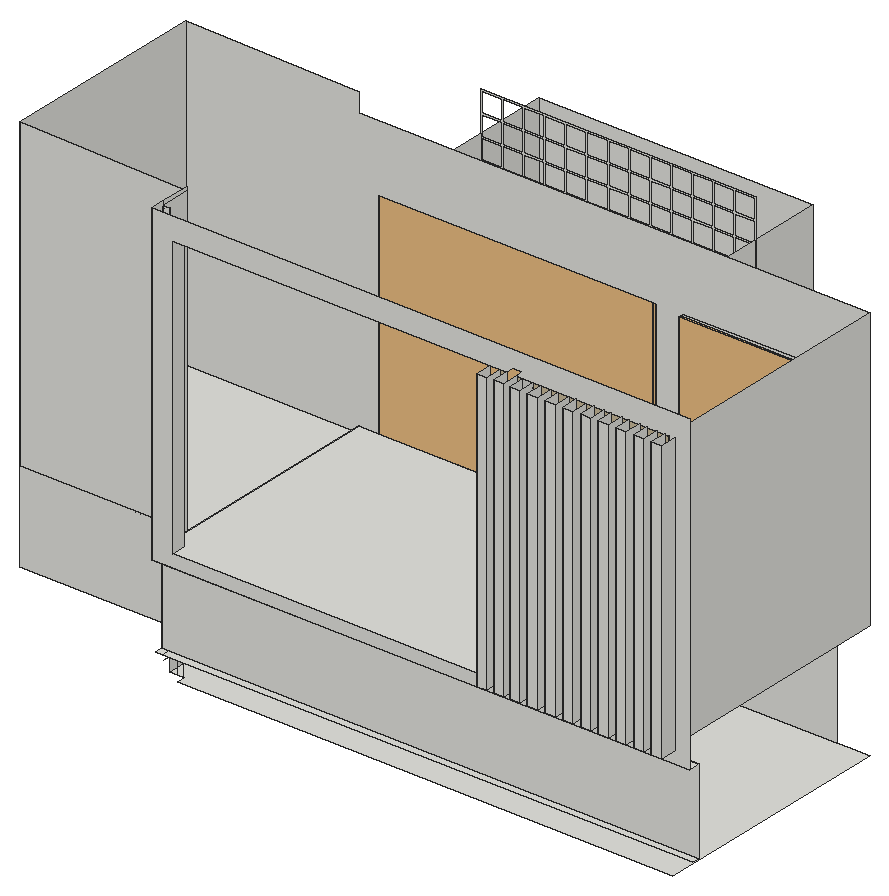
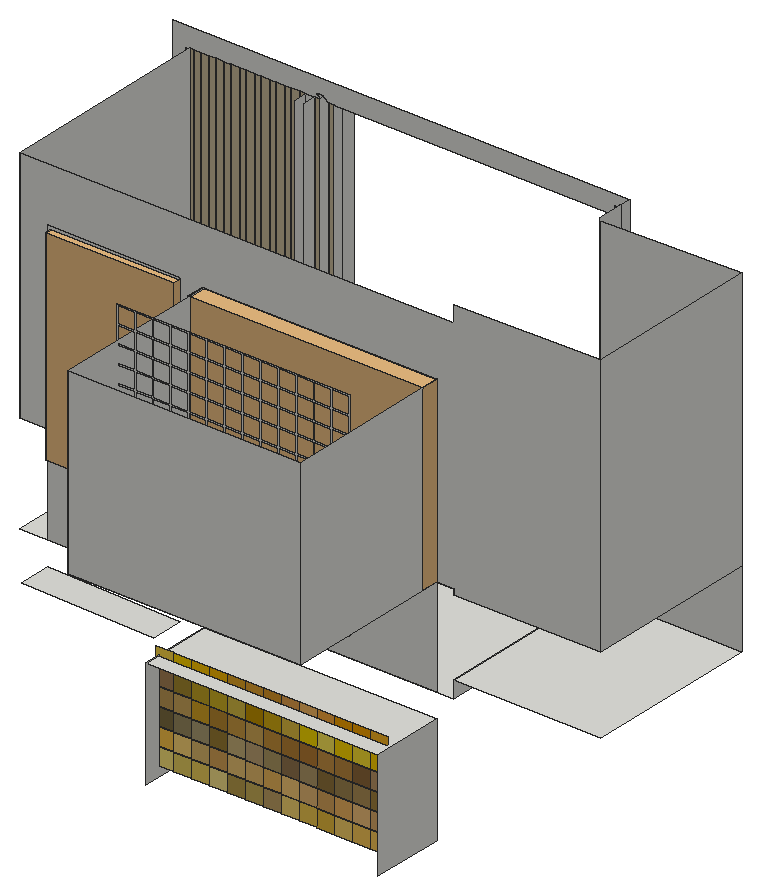
# SketchUp Ruby script. Lengths in inches.
U = 1.inch
M = Sketchup.active_model
def pt(a) = Geom::Point3d.new(a.map { |v| v * U })
def face(e, loops, mat)
  f = e.add_face(loops[0].map { |a| pt(a) })
  loops[1..].each { |l| e.add_face(l.map { |a| pt(a) }).erase! }
  f.material = f.back_material = mat if mat
  f
end
# faces: each face lists its corners as indices into pts; further lists are holes
def faces(e, pts, list, mat = nil) = list.each { |f| face(e, (f[0].is_a?(Array) ? f : [f]).map { |l| l.map { |i| pts[i] } }, mat) }
# xy, xz, yz: faces in a plane at the given z, y or x. An outline is a flat list of corners, or four numbers for a rectangle; further outlines are holes
def ring(l) = l.size == 4 ? [[l[0], l[1]], [l[2], l[1]], [l[2], l[3]], [l[0], l[3]]] : l.each_slice(2).to_a
def flat(e, list, mat, &to3) = list.each { |f| face(e, (f[0].is_a?(Array) ? f : [f]).map { |l| ring(l).map { |u, v| to3.(u, v) } }, mat) }
def xy(e, z, list, mat = nil) = flat(e, list, mat) { |x, y| [x, y, z] }
def xz(e, y, list, mat = nil) = flat(e, list, mat) { |x, z| [x, y, z] }
def yz(e, x, list, mat = nil) = flat(e, list, mat) { |y, z| [x, y, z] }
def lines(e, pts, list) = list.each { |a, b| e.add_line(pt(pts[a]), pt(pts[b])) }
# prism: a flat outline (further loops are holes) pulled along v
def prism(e, loops, v, mat = nil)
  f = face(e, loops, mat); d = Geom::Vector3d.new(v.map { |x| x * U })
  f.pushpull(f.normal.samedirection?(d) ? d.length : -d.length)
end
def box(e, o, s, mat = nil) = prism(e, [[o, [o[0] + s[0], o[1], o[2]], [o[0] + s[0], o[1] + s[1], o[2]], [o[0], o[1] + s[1], o[2]]]], [0, 0, s[2]], mat)
def at(x, y, z, deg = 0) = Geom::Transformation.translation(pt([x, y, z])) * Geom::Transformation.rotation(ORIGIN, Z_AXIS, deg.degrees)
def axes(o, x, y, z) = Geom::Transformation.new([*x, 0, *y, 0, *z, 0, *pt(o).to_a, 1])
def part(name) = M.definitions.add(name)
# library, detail: a bought-in or finely detailed component or shape, given as its bounding box
def library(name, o, s) = part(name).tap { |d| box(d.entities, o, s) }
def detail(e, o, s) = box(e.add_group.entities, o, s)
def put(e, d, t, mat = nil) = e.add_instance(d, t).tap { |i| i.material = mat if mat }
def group(e, t, mat = nil) = e.add_group.tap { |g| g.transformation = t; g.material = mat if mat }.entities
root = M.entities
M.materials.add("SW 0028 Caen Stone").color = [234, 212, 175]
M.materials.add("SW 0043 Peristyle Brass").color = [171, 151, 98]
M.materials.add("SW 2813 Downing Straw").color = [196, 173, 119]
M.materials.add("SW 2814 Rookwood Antique Gold").color = [158, 131, 78]
M.materials.add("SW 2817 Rookwood Amber").color = [185, 135, 62]
M.materials.add("SW 2831 Classical Gold").color = [230, 191, 112]
M.materials.add("SW 2858 Harvest Gold").color = [215, 167, 103]
M.materials.add("SW 6113 Interactive Cream").color = [226, 206, 173]
M.materials.add("SW 6116 Tatami Tan").color = [184, 148, 100]
M.materials.add("SW 6117 Smokey Topaz").color = [164, 127, 83]
M.materials.add("SW 6118 Leather Bound").color = [139, 102, 57]
M.materials.add("SW 6120 Believable Buff").color = [216, 202, 167]
M.materials.add("SW 6123 Baguette").color = [175, 151, 103]
M.materials.add("SW 6127 Ivoire").color = [224, 209, 170]
M.materials.add("SW 6130 Mannered Gold").color = [189, 159, 99]
M.materials.add("SW 6131 Chamois").color = [172, 141, 84]
M.materials.add("SW 6132 Relic Bronze").color = [143, 113, 59]
M.materials.add("SW 6134 Netsuke").color = [220, 210, 175]
M.materials.add("SW 6137 Burlap").color = [170, 155, 114]
M.materials.add("SW 6138 Artifact").color = [151, 136, 95]
M.materials.add("SW 6139 Mossy Gold").color = [124, 107, 64]
M.materials.add("SW 6365 Cachet Cream").color = [240, 220, 183]
M.materials.add("SW 6367 Viva Gold").color = [227, 182, 114]
M.materials.add("SW 6368 Bakelite Gold").color = [212, 162, 89]
M.materials.add("SW 6369 Tassel").color = [195, 143, 67]
M.materials.add("SW 6370 Saucy Gold").color = [179, 122, 51]
M.materials.add("SW 6372 Inviting Ivory").color = [239, 218, 175]
M.materials.add("SW 6374 Torchlight").color = [226, 185, 106]
M.materials.add("SW 6375 Honeycomb").color = [210, 161, 84]
M.materials.add("SW 6376 Gold Coast").color = [195, 143, 57]
M.materials.add("SW 6377 Butterscotch").color = [180, 128, 52]
M.materials.add("SW 6379 Jersey Cream").color = [239, 224, 185]
M.materials.add("SW 6381 Anjou Pear").color = [217, 181, 105]
M.materials.add("SW 6382 Ceremonial Gold").color = [208, 167, 85]
M.materials.add("SW 6383 Golden Rule").color = [199, 153, 65]
M.materials.add("SW 6384 Cut The Mustard").color = [182, 135, 47]
M.materials.add("SW 6387 Compatible Cream").color = [229, 206, 156]
M.materials.add("SW 6389 Butternut").color = [200, 164, 90]
M.materials.add("SW 6390 Bosc Pear").color = [188, 151, 83]
M.materials.add("SW 6391 Gallant Gold").color = [161, 128, 61]
M.materials.add("SW 6393 Convivial Yellow").color = [229, 218, 173]
M.materials.add("SW 6395 Alchemy").color = [197, 171, 86]
M.materials.add("SW 6396 Different Gold").color = [183, 156, 75]
M.materials.add("SW 6397 Nankeen").color = [162, 135, 46]
M.materials.add("SW 6398 Sconce Gold").color = [151, 121, 51]
M.materials.add("SW 6400 Lucent Yellow").color = [223, 213, 164]
M.materials.add("SW 6407 Ancestral Gold").color = [218, 210, 164]
M.materials.add("SW 6661 Papaya").color = [238, 189, 120]
M.materials.add("SW 6662 Summer Day").color = [234, 176, 94]
M.materials.add("SW 6663 Saffron Thread").color = [223, 158, 74]
M.materials.add("SW 6668 Sunrise").color = [242, 197, 116]
M.materials.add("SW 6669 Yarrow").color = [231, 180, 89]
M.materials.add("SW 6670 Gold Crest").color = [221, 159, 46]
M.materials.add("SW 6671 Curry").color = [214, 148, 38]
M.materials.add("SW 6675 Afternoon").color = [248, 209, 116]
M.materials.add("SW 6676 Butterfield").color = [244, 196, 86]
M.materials.add("SW 6677 Goldenrod").color = [244, 196, 86]
M.materials.add("SW 6678 Sunflower").color = [223, 162, 35]
M.materials.add("SW 6682 June Day").color = [242, 210, 111]
M.materials.add("SW 6683 Bee").color = [235, 196, 79]
M.materials.add("SW 6684 Brittlebush").color = [228, 184, 61]
M.materials.add("SW 6685 Trinket").color = [209, 161, 37]
M.materials.add("SW 6689 Overjoy").color = [233, 203, 89]
M.materials.add("SW 6690 Gambol Gold").color = [220, 186, 63]
M.materials.add("SW 6691 Glitzy Gold").color = [208, 168, 18]
M.materials.add("SW 6692 Auric").color = [191, 145, 0]
M.materials.add("SW 6695 Midday").color = [242, 222, 135]
M.materials.add("SW 6696 Quilt Gold").color = [227, 203, 95]
M.materials.add("SW 6697 Nugget").color = [211, 184, 67]
M.materials.add("SW 6698 Kingdom Gold").color = [202, 173, 37]
M.materials.add("SW 6699 Crispy Gold").color = [191, 161, 37]
M.materials.add("SW 6701 Moonraker").color = [234, 231, 176]
M.materials.add("SW 6889 Stirring Orange").color = [243, 181, 96]
M.materials.add("SW 6890 Osage Orange").color = [243, 166, 60]
M.materials.add("SW 6894 Forceful Orange").color = [242, 160, 0]
M.materials.add("SW 6895 Laughing Orange").color = [242, 160, 0]
M.materials.add("SW 6897 Sundance").color = [245, 206, 103]
M.materials.add("SW 6898 Social Butterfly").color = [247, 193, 71]
M.materials.add("SW 6899 Nasturtiumb").color = [246, 178, 33]
M.materials.add("SW 6901 Daffodil").color = [246, 223, 119]
M.materials.add("SW 6902 Decisive Yellow").color = [248, 211, 68]
M.materials.add("SW 6903 Cheerful").color = [250, 208, 0]
M.materials.add("SW 6904 Gusto Gold").color = [245, 181, 0]
M.materials.add("SW 6905 Goldfinch").color = [249, 192, 0]
M.materials.add("SW 6906 Citrus").color = [251, 205, 0]
M.materials.add("SW 6907 Forsythia").color = [251, 210, 0]
M.materials.add("SW 6909 Lemon Twist").color = [248, 227, 86]
M.materials.add("SW 6910 Daisy").color = [246, 220, 49]
M.materials.add("SW 6911 Confident Yellow").color = [245, 214, 0]
M.materials.add("SW 7537 Irish Cream").color = [227, 211, 186]
M.materials.add("SW 7676 Paper Lantern").color = [240, 224, 198]
M.materials.add("SW 7678 Cottage Cream").color = [236, 219, 189]
M.materials.add("SW 7681 Tea Light").color = [246, 227, 194]
M.materials.add("SW 7683 Buff").color = [242, 225, 197]
M.materials.add("SW 7684 Concord Buff").color = [239, 216, 182]
M.materials.add("SW 7686 Hinoki").color = [246, 220, 183]
M.materials.add("SW 7687 August Moon").color = [231, 199, 161]
M.materials.add("SW 7688 Sundew").color = [223, 206, 176]
M.materials.add("SW 7696 Toasted Pine Nut").color = [218, 199, 167]
M.materials.add("SW 7698 Straw Harvest").color = [217, 199, 161]
M.materials.add("SW 7699 Rustic City").color = [188, 160, 113]
M.materials.add("SW 7700 Olde World Gold").color = [145, 116, 76]
M.materials.add("[Quartz Light Brown]").color = [199, 184, 152]
c1 = library("Group6\#1",[-22.44,-5.97,0],[42.52,9.29,84.25])
c2 = library("Glass_door",[70.54,1.5625,0],[78.74,7.87,82.68])
xy(root,1139.55,[[1349.53,376.08,1604.22,455.83]])
xy(root,1165.72,[[1344.39,147.66,1344.39,155.91,1330.95,155.91,1330.95,376.08,1805.83,376.08,1805.83,147.66]])
xy(root,1184.06,[[1324.51,147.66,1330.95,154.6],[1330.95,147.66,1824.45,154.6],[1324.16,154.6,1324.51,155.91],[1324.51,154.6,1330.95,155.91],[1330.44,155.91,1330.44,183.72,1169.07,183.72,1169.07,376.08,1330.95,376.08,1330.95,155.91],
  [1324.51,155.91,1330.44,183.72]])
xy(root,1262.78,[[1324.16,143.16,1824.45,154.6]])
xy(root,1268.3125,[[1324.16,155.91,1324.51,183.72],[1324.51,155.91,1330.44,183.72],[1169.07,183.72,1324.16,376.08],[1324.16,183.72,1330.44,376.08]])
xy(root,1274.1875,[[1638.86,127.85,1648.04,143.16],[1654.29,127.85,1663.98,143.16],[1669.29,127.85,1678.97,143.16],[1343.63,143.16,1669.29,143.16,1669.29,158.47,1678.97,158.47,1678.97,143.16,1805.83,143.16,1805.83,376.08,1330.44,376.08,1330.44,155.91,1343.63,155.91],[1669.29,143.16,1678.97,158.47],
  [1349.53,376.08,1604.22,561.95]])
xz(root,127.85,[[1638.86,1274.1875,1648.04,1534.95],[1654.29,1274.1875,1663.98,1534.95],[1669.29,1274.1875,1678.97,1534.95],[1685.79,1274.1875,1695.47,1534.95],[1702.29,1274.1875,1711.97,1534.95],
  [1718.79,1274.1875,1728.47,1534.95],[1735.29,1274.1875,1744.97,1534.95],[1751.79,1274.1875,1761.47,1534.95],[1768.29,1274.1875,1777.97,1534.95],[1784.79,1274.1875,1794.47,1534.95],
  [1801.29,1274.1875,1810.97,1534.95]])
xz(root,143.16,[[[1324.16,1262.78,1824.45,1555.875],[1343.63,1274.1875,1343.63,1534.95,1654.29,1534.95,1659.92,1540.4375,1669.6,1540.4375,1663.98,1534.95,1805.83,1534.95,1805.83,1274.1875]]])
xz(root,143.16,[[1648.04,1274.1875,1654.29,1534.95],[1663.98,1274.1875,1669.29,1534.95],[1678.97,1274.1875,1685.79,1534.95],[1685.79,1274.1875,1695.47,1534.95],[1695.47,1274.1875,1702.29,1534.95],
  [1702.29,1274.1875,1711.97,1534.95],[1711.97,1274.1875,1718.79,1534.95],[1718.79,1274.1875,1728.47,1534.95],[1728.47,1274.1875,1735.29,1534.95],[1735.29,1274.1875,1744.97,1534.95],
  [1744.97,1274.1875,1751.79,1534.95],[1751.79,1274.1875,1761.47,1534.95],[1761.47,1274.1875,1768.29,1534.95],[1768.29,1274.1875,1777.97,1534.95],[1777.97,1274.1875,1784.79,1534.95],
  [1784.79,1274.1875,1794.47,1534.95],[1794.47,1274.1875,1801.29,1534.95],[1801.29,1274.1875,1805.83,1534.95]],"[Quartz Light Brown]")
xz(root,154.6,[[1324.16,1184.06,1824.45,1262.78]])
xz(root,155.91,[[1324.16,1184.06,1324.61,1268.3125],[1324.61,1184.06,1329.57,1268.3125],[1329.57,1184.06,1330.44,1268.3125],[1324.16,1268.3125,1324.51,1555.875],[1324.51,1268.3125,1324.61,1552.52],
  [1324.61,1268.3125,1329.57,1552.52],[1329.57,1268.3125,1329.57,1552.52,1330.44,1552.52,1330.44,1534.95,1337.99,1534.95,1337.99,1274.1875,1330.44,1274.1875,1330.44,1268.3125],[1337.99,1274.1875,1342.94,1534.95],[1342.94,1274.1875,1343.63,1534.95]])
xz(root,183.72,[[1169.07,1184.06,1330.44,1268.3125],[1169.07,1268.3125,1169.07,1555.64,1324.16,1552.64,1324.16,1268.3125],[1324.16,1268.3125,1324.16,1552.64,1324.51,1552.63,1324.51,1268.3125]])
xz(root,376.08,[[1349.53,1165.72,1604.22,1274.1875],[1604.22,1165.72,1630.81,1274.1875],[1630.81,1165.72,1775.37,1274.1875],[1169.07,1268.3125,1330.44,1268.3125,1330.44,1274.1875,1349.53,1274.1875,1349.53,1472.71,1604.22,1472.71,1604.22,1274.1875,1630.81,1274.1875,1630.81,1473,1775.37,1474.54,1775.37,1274.1875,1805.83,1274.1875,1805.83,1534.95,1330.44,1534.95,1330.44,1552.52,1169.07,1555.64],[1630.81,1274.1875,1775.37,1274.1875,1775.37,1474.54,1630.81,1473]])
xz(root,438.51,[[1470.29,1071,1488.94,1089.65]],"SW 0043 Peristyle Brass")
xz(root,438.51,[[1509.5,1071,1528.15,1089.65]],"SW 2813 Downing Straw")
xz(root,438.51,[[1391.88,1071,1410.54,1089.65]],"SW 2814 Rookwood Antique Gold")
xz(root,438.51,[[1391.88,1090.6,1410.54,1109.25]],"SW 2817 Rookwood Amber")
xz(root,438.51,[[1509.5,1051.4,1528.15,1070.05]],"SW 2831 Classical Gold")
xz(root,438.51,[[1352.68,1051.4,1371.33,1070.05]],"SW 2858 Harvest Gold")
xz(root,438.51,[[1352.68,1090.6,1371.33,1109.25]],"SW 6116 Tatami Tan")
xz(root,438.51,[[1587.9,1110.2,1606.56,1128.86]],"SW 6117 Smokey Topaz")
xz(root,438.51,[[1372.28,1090.6,1390.93,1109.25]],"SW 6118 Leather Bound")
xz(root,438.51,[[1431.09,1071,1449.74,1089.65]],"SW 6123 Baguette")
xz(root,438.51,[[1470.29,1031.8,1488.94,1050.45]],"SW 6130 Mannered Gold")
xz(root,438.51,[[1372.28,1071,1390.93,1089.65]],"SW 6131 Chamois")
xz(root,438.51,[[1411.49,1071,1430.14,1089.65]],"SW 6132 Relic Bronze")
xz(root,438.51,[[1548.7,1071,1567.35,1089.65]],"SW 6137 Burlap")
xz(root,438.51,[[1568.3,1071,1586.95,1089.65]],"SW 6138 Artifact")
xz(root,438.51,[[1587.9,1071,1606.56,1089.65]],"SW 6139 Mossy Gold")
xz(root,438.51,[[1431.09,1051.4,1449.74,1070.05]],"SW 6367 Viva Gold")
xz(root,438.51,[[1411.49,1051.4,1430.14,1070.05]],"SW 6368 Bakelite Gold")
xz(root,438.51,[[1411.49,1090.6,1430.14,1109.25]],"SW 6369 Tassel")
xz(root,438.51,[[1431.09,1090.6,1449.74,1109.25]],"SW 6370 Saucy Gold")
xz(root,438.51,[[1489.89,1051.4,1508.55,1070.05]],"SW 6374 Torchlight")
xz(root,438.51,[[1529.1,1051.4,1547.75,1070.05]],"SW 6375 Honeycomb")
xz(root,438.51,[[1470.29,1090.6,1488.94,1109.25]],"SW 6376 Gold Coast")
xz(root,438.51,[[1450.69,1090.6,1469.34,1109.25]],"SW 6377 Butterscotch")
xz(root,438.51,[[1548.7,1051.4,1567.35,1070.05]],"SW 6381 Anjou Pear")
xz(root,438.51,[[1489.89,1090.6,1508.55,1109.25]],"SW 6382 Ceremonial Gold")
xz(root,438.51,[[1509.5,1090.6,1528.15,1109.25]],"SW 6383 Golden Rule")
xz(root,438.51,[[1529.1,1090.6,1547.75,1109.25]],"SW 6384 Cut The Mustard")
xz(root,438.51,[[1568.3,1090.6,1586.95,1109.25]],"SW 6389 Butternut")
xz(root,438.51,[[1587.9,1090.6,1606.56,1109.25]],"SW 6390 Bosc Pear")
xz(root,438.51,[[1352.68,1071,1371.33,1089.65]],"SW 6391 Gallant Gold")
xz(root,438.51,[[1489.89,1031.8,1508.55,1050.45]],"SW 6395 Alchemy")
xz(root,438.51,[[1509.5,1031.8,1528.15,1050.45]],"SW 6396 Different Gold")
xz(root,438.51,[[1568.3,1110.2,1586.95,1128.86]],"SW 6397 Nankeen")
xz(root,438.51,[[1529.1,1071,1547.75,1089.65]],"SW 6398 Sconce Gold")
xz(root,438.51,[[1372.28,1051.4,1390.93,1070.05]],"SW 6661 Papaya")
xz(root,438.51,[[1391.88,1051.4,1410.54,1070.05]],"SW 6662 Summer Day")
xz(root,438.51,[[1450.69,1129.81,1469.34,1148.46]],"SW 6663 Saffron Thread")
xz(root,438.51,[[1450.69,1051.4,1469.34,1070.05]],"SW 6668 Sunrise")
xz(root,438.51,[[1470.29,1051.4,1488.94,1070.05]],"SW 6669 Yarrow")
xz(root,438.51,[[1489.89,1129.81,1508.55,1148.46]],"SW 6670 Gold Crest")
xz(root,438.51,[[1470.29,1129.81,1488.94,1148.46]],"SW 6671 Curry")
xz(root,438.51,[[1568.3,1051.4,1586.95,1070.05]],"SW 6675 Afternoon")
xz(root,438.51,[[1352.68,1031.8,1371.33,1050.45]],"SW 6676 Butterfield")
xz(root,438.51,[[1372.28,1031.8,1390.93,1050.45]],"SW 6677 Goldenrod")
xz(root,438.51,[[1509.5,1129.81,1528.15,1148.46]],"SW 6678 Sunflower")
xz(root,438.51,[[1450.69,1031.8,1469.34,1050.45]],"SW 6682 June Day")
xz(root,438.51,[[1431.09,1031.8,1449.74,1050.45]],"SW 6683 Bee")
xz(root,438.51,[[1411.49,1031.8,1430.14,1050.45]],"SW 6684 Brittlebush")
xz(root,438.51,[[1548.7,1090.6,1567.35,1109.25]],"SW 6685 Trinket")
xz(root,438.51,[[1548.7,1031.8,1567.35,1050.45]],"SW 6689 Overjoy")
xz(root,438.51,[[1450.69,1110.2,1469.34,1128.86]],"SW 6690 Gambol Gold")
xz(root,438.51,[[1470.29,1110.2,1488.94,1128.86]],"SW 6691 Glitzy Gold")
xz(root,438.51,[[1489.89,1110.2,1508.55,1128.86]],"SW 6692 Auric")
xz(root,438.51,[[1529.1,1031.8,1547.75,1050.45]],"SW 6695 Midday")
xz(root,438.51,[[1568.3,1031.8,1586.95,1050.45]],"SW 6696 Quilt Gold")
xz(root,438.51,[[1509.5,1110.2,1528.15,1128.86]],"SW 6697 Nugget")
xz(root,438.51,[[1529.1,1110.2,1547.75,1128.86]],"SW 6698 Kingdom Gold")
xz(root,438.51,[[1548.7,1110.2,1567.35,1128.86]],"SW 6699 Crispy Gold")
xz(root,438.51,[[1431.09,1129.81,1449.74,1148.46]],"SW 6889 Stirring Orange")
xz(root,438.51,[[1411.49,1129.81,1430.14,1148.46]],"SW 6890 Osage Orange")
xz(root,438.51,[[1391.88,1129.81,1410.54,1148.46]],"SW 6894 Forceful Orange")
xz(root,438.51,[[1372.28,1129.81,1390.93,1148.46]],"SW 6895 Laughing Orange")
xz(root,438.51,[[1391.88,1031.8,1410.54,1050.45]],"SW 6897 Sundance")
xz(root,438.51,[[1587.9,1051.4,1606.56,1070.05]],"SW 6898 Social Butterfly")
xz(root,438.51,[[1352.68,1129.81,1371.33,1148.46]],"SW 6899 Nasturtiumb")
xz(root,438.51,[[1587.9,1031.8,1606.56,1050.45]],"SW 6901 Daffodil")
xz(root,438.51,[[1587.9,1129.81,1606.56,1148.46]],"SW 6902 Decisive Yellow")
xz(root,438.51,[[1568.3,1129.81,1586.95,1148.46]],"SW 6903 Cheerful")
xz(root,438.51,[[1529.1,1129.81,1547.75,1148.46]],"SW 6904 Gusto Gold")
xz(root,438.51,[[1548.7,1129.81,1567.35,1148.46]],"SW 6905 Goldfinch")
xz(root,438.51,[[1352.68,1110.2,1371.33,1128.86]],"SW 6906 Citrus")
xz(root,438.51,[[1391.88,1110.2,1410.54,1128.86]],"SW 6907 Forsythia")
xz(root,438.51,[[1411.49,1110.2,1430.14,1128.86]],"SW 6909 Lemon Twist")
xz(root,438.51,[[1372.28,1110.2,1390.93,1128.86]],"SW 6910 Daisy")
xz(root,438.51,[[1431.09,1110.2,1449.74,1128.86]],"SW 6911 Confident Yellow")
xz(root,438.51,[[1489.89,1071,1508.55,1089.65]],"SW 7699 Rustic City")
xz(root,438.51,[[1450.69,1071,1469.34,1089.65]],"SW 7700 Olde World Gold")
xz(root,494.58,[[[1349.39,1273.24,1605.17,1509.41],[1585.57,1391.8,1604.22,1410.45],[1350.34,1391.8,1369,1410.45],[1369.95,1391.8,1388.6,1410.45],[1389.55,1391.8,1408.2,1410.45],[1409.15,1391.8,1427.8,1410.45],[1428.75,1391.8,1447.4,1410.45],[1448.35,1391.8,1467.01,1410.45],[1467.96,1391.8,1486.61,1410.45],[1487.56,1391.8,1506.21,1410.45],[1507.16,1391.8,1525.8125,1410.45],[1526.76,1391.8,1545.41,1410.45],[1546.36,1391.8,1565.02,1410.45],[1565.97,1391.8,1584.62,1410.45],[1585.57,1372.2,1604.22,1390.85],[1350.34,1372.2,1369,1390.85],[1369.95,1372.2,1388.6,1390.85],[1389.55,1372.2,1408.2,1390.85],[1409.15,1372.2,1427.8,1390.85],[1428.75,1372.2,1447.4,1390.85],[1448.35,1372.2,1467.01,1390.85],[1467.96,1372.2,1486.61,1390.85],[1487.56,1372.2,1506.21,1390.85],[1507.16,1372.2,1525.8125,1390.85],[1526.76,1372.2,1545.41,1390.85],[1546.36,1372.2,1565.02,1390.85],[1565.97,1372.2,1584.62,1390.85],[1585.57,1352.6,1604.22,1371.25],[1585.57,1411.4,1604.22,1430.05],[1585.57,1431,1604.22,1449.66],[1585.57,1450.61,1604.22,1469.26],[1585.57,1470.21,1604.22,1488.86],[1585.57,1274.1875,1604.22,1292.84],[1585.57,1313.39,1604.22,1332.04],[1350.34,1470.21,1369,1488.86],[1350.34,1450.61,1369,1469.26],[1350.34,1431,1369,1449.66],[1350.34,1411.4,1369,1430.05],[1350.34,1352.6,1369,1371.25],[1369.95,1470.21,1388.6,1488.86],[1369.95,1450.61,1388.6,1469.26],[1369.95,1431,1388.6,1449.66],[1369.95,1411.4,1388.6,1430.05],[1369.95,1352.6,1388.6,1371.25],[1389.55,1352.6,1408.2,1371.25],[1389.55,1411.4,1408.2,1430.05],[1389.55,1431,1408.2,1449.66],[1389.55,1450.61,1408.2,1469.26],[1389.55,1470.21,1408.2,1488.86],[1409.15,1352.6,1427.8,1371.25],[1409.15,1411.4,1427.8,1430.05],[1409.15,1431,1427.8,1449.66],[1409.15,1450.61,1427.8,1469.26],[1409.15,1470.21,1427.8,1488.86],[1585.57,1293.79,1604.22,1312.44],[1350.34,1274.1875,1369,1292.84],[1369.95,1274.1875,1388.6,1292.84],[1389.55,1274.1875,1408.2,1292.84],[1409.15,1274.1875,1427.8,1292.84],[1428.75,1411.4,1447.4,1430.05],[1428.75,1352.6,1447.4,1371.25],[1428.75,1450.61,1447.4,1469.26],[1428.75,1470.21,1447.4,1488.86],[1428.75,1431,1447.4,1449.66],[1448.35,1470.21,1467.01,1488.86],[1448.35,1450.61,1467.01,1469.26],[1448.35,1431,1467.01,1449.66],[1448.35,1411.4,1467.01,1430.05],[1448.35,1352.6,1467.01,1371.25],[1467.96,1470.21,1486.61,1488.86],[1467.96,1450.61,1486.61,1469.26],[1467.96,1352.6,1486.61,1371.25],[1467.96,1411.4,1486.61,1430.05],[1467.96,1431,1486.61,1449.66],[1487.56,1352.6,1506.21,1371.25],[1487.56,1411.4,1506.21,1430.05],[1487.56,1431,1506.21,1449.66],[1487.56,1450.61,1506.21,1469.26],[1487.56,1470.21,1506.21,1488.86],[1507.16,1352.6,1525.8125,1371.25],[1507.16,1411.4,1525.8125,1430.05],[1507.16,1431,1525.8125,1449.66],[1507.16,1450.61,1525.8125,1469.26],[1507.16,1470.21,1525.8125,1488.86],[1526.76,1352.6,1545.41,1371.25],[1526.76,1411.4,1545.41,1430.05],[1526.76,1431,1545.41,1449.66],[1526.76,1450.61,1545.41,1469.26],[1526.76,1470.21,1545.41,1488.86],[1546.36,1352.6,1565.02,1371.25],[1546.36,1411.4,1565.02,1430.05],[1546.36,1431,1565.02,1449.66],[1546.36,1450.61,1565.02,1469.26],[1546.36,1470.21,1565.02,1488.86],[1565.97,1352.6,1584.62,1371.25],[1565.97,1411.4,1584.62,1430.05],[1565.97,1431,1584.62,1449.66],[1565.97,1450.61,1584.62,1469.26],[1565.97,1470.21,1584.62,1488.86],[1350.34,1313.39,1369,1332.04],[1369.95,1313.39,1388.6,1332.04],[1389.55,1313.39,1408.2,1332.04],[1409.15,1313.39,1427.8,1332.04],[1428.75,1274.1875,1447.4,1292.84],[1448.35,1274.1875,1467.01,1292.84],[1467.96,1274.1875,1486.61,1292.84],[1487.56,1274.1875,1506.21,1292.84],[1507.16,1274.1875,1525.8125,1292.84],[1526.76,1274.1875,1545.41,1292.84],[1546.36,1274.1875,1565.02,1292.84],[1565.97,1274.1875,1584.62,1292.84],[1350.34,1293.79,1369,1312.44],[1369.95,1293.79,1388.6,1312.44],[1389.55,1293.79,1408.2,1312.44],[1409.15,1293.79,1427.8,1312.44],[1428.75,1313.39,1447.4,1332.04],[1448.35,1313.39,1467.01,1332.04],[1467.96,1313.39,1486.61,1332.04],[1487.56,1313.39,1506.21,1332.04],[1507.16,1313.39,1525.8125,1332.04],[1526.76,1313.39,1545.41,1332.04],[1546.36,1313.39,1565.02,1332.04],[1565.97,1313.39,1584.62,1332.04],[1428.75,1293.79,1447.4,1312.44],[1448.35,1293.79,1467.01,1312.44],[1467.96,1293.79,1486.61,1312.44],[1487.56,1293.79,1506.21,1312.44],[1507.16,1293.79,1525.8125,1312.44],[1526.76,1293.79,1545.41,1312.44],[1546.36,1293.79,1565.02,1312.44],[1565.97,1293.79,1584.62,1312.44],[1585.57,1489.81,1604.22,1508.46],[1585.57,1332.99,1604.22,1351.65],[1350.34,1489.81,1369,1508.46],[1350.34,1332.99,1369,1351.65],[1369.95,1332.99,1388.6,1351.65],[1369.95,1489.81,1388.6,1508.46],[1389.55,1489.81,1408.2,1508.46],[1389.55,1332.99,1408.2,1351.65],[1409.15,1489.81,1427.8,1508.46],[1409.15,1332.99,1427.8,1351.65],[1428.75,1332.99,1447.4,1351.65],[1428.75,1489.81,1447.4,1508.46],[1448.35,1332.99,1467.01,1351.65],[1448.35,1489.81,1467.01,1508.46],[1467.96,1489.81,1486.61,1508.46],[1467.96,1332.99,1486.61,1351.65],[1487.56,1489.81,1506.21,1508.46],[1487.56,1332.99,1506.21,1351.65],[1507.16,1489.81,1525.8125,1508.46],[1507.16,1332.99,1525.8125,1351.65],[1526.76,1489.81,1545.41,1508.46],[1526.76,1332.99,1545.41,1351.65],[1546.36,1489.81,1565.02,1508.46],[1546.36,1332.99,1565.02,1351.65],[1565.97,1489.81,1584.62,1508.46],[1565.97,1332.99,1584.62,1351.65]],[1565.97,1274.1875,1584.62,1292.84],[1585.57,1274.1875,1604.22,1292.84]])
xz(root,494.58,[[1369.95,1293.79,1388.6,1312.44]],"SW 0028 Caen Stone")
xz(root,494.58,[[1409.15,1293.79,1427.8,1312.44]],"SW 6113 Interactive Cream")
xz(root,494.58,[[1448.35,1274.1875,1467.01,1292.84]],"SW 6120 Believable Buff")
xz(root,494.58,[[1409.15,1274.1875,1427.8,1292.84]],"SW 6127 Ivoire")
xz(root,494.58,[[1467.96,1274.1875,1486.61,1292.84]],"SW 6134 Netsuke")
xz(root,494.58,[[1389.55,1293.79,1408.2,1312.44]],"SW 6365 Cachet Cream")
xz(root,494.58,[[1507.16,1293.79,1525.8125,1312.44]],"SW 6372 Inviting Ivory")
xz(root,494.58,[[1565.97,1293.79,1584.62,1312.44]],"SW 6379 Jersey Cream")
xz(root,494.58,[[1350.34,1274.1875,1369,1292.84]],"SW 6387 Compatible Cream")
xz(root,494.58,[[1487.56,1274.1875,1506.21,1292.84]],"SW 6393 Convivial Yellow")
xz(root,494.58,[[1526.76,1274.1875,1545.41,1292.84]],"SW 6400 Lucent Yellow")
xz(root,494.58,[[1546.36,1274.1875,1565.02,1292.84]],"SW 6407 Ancestral Gold")
xz(root,494.58,[[1350.34,1293.79,1369,1312.44]],"SW 6701 Moonraker")
xz(root,494.58,[[1428.75,1293.79,1447.4,1312.44]],"SW 7537 Irish Cream")
xz(root,494.58,[[1526.76,1293.79,1545.41,1312.44]],"SW 7676 Paper Lantern")
xz(root,494.58,[[1389.55,1274.1875,1408.2,1292.84]],"SW 7678 Cottage Cream")
xz(root,494.58,[[1487.56,1293.79,1506.21,1312.44]],"SW 7681 Tea Light")
xz(root,494.58,[[1467.96,1293.79,1486.61,1312.44]],"SW 7683 Buff")
xz(root,494.58,[[1369.95,1274.1875,1388.6,1292.84]],"SW 7684 Concord Buff")
xz(root,494.58,[[1585.57,1293.79,1604.22,1312.44]],"SW 7686 Hinoki")
xz(root,494.58,[[1546.36,1293.79,1565.02,1312.44]],"SW 7687 August Moon")
xz(root,494.58,[[1448.35,1293.79,1467.01,1312.44]],"SW 7688 Sundew")
xz(root,494.58,[[1428.75,1274.1875,1447.4,1292.84]],"SW 7696 Toasted Pine Nut")
xz(root,494.58,[[1507.16,1274.1875,1525.8125,1292.84]],"SW 7698 Straw Harvest")
xz(root,561.95,[[1349.53,1274.1875,1604.22,1472.71]])
yz(root,1169.07,[[183.72,1268.3125,376.08,1555.64]])
yz(root,1324.16,[[154.6,1184.06,154.6,1262.78,143.16,1262.78,143.16,1555.875,155.91,1555.875,155.91,1184.06],[155.91,1268.3125,183.72,1555.875]])
yz(root,1324.51,[[155.91,1268.3125,183.72,1552.52]])
yz(root,1330.44,[[155.91,1184.06,183.72,1268.3125],[155.91,1268.3125,183.72,1274.1875],[183.72,1268.3125,376.08,1274.1875]])
yz(root,1330.95,[[155.91,1165.72,376.08,1184.06]])
yz(root,1343.63,[[143.16,1274.1875,155.91,1534.95]])
yz(root,1349.53,[[376.08,1019.96,455.83,1139.55],[376.08,1274.1875,561.95,1472.71]])
yz(root,1604.22,[[376.08,1019.96,455.83,1139.55],[376.08,1274.1875,561.95,1472.71]])
yz(root,1638.86,[[127.85,1274.1875,143.16,1534.95]])
yz(root,1648.04,[[127.85,1274.1875,143.16,1534.95]])
yz(root,1654.29,[[127.85,1274.1875,143.16,1534.95]])
yz(root,1663.98,[[127.85,1274.1875,143.16,1534.95]])
yz(root,1669.29,[[127.85,1274.1875,143.16,1534.95],[143.16,1274.1875,158.47,1534.95]])
yz(root,1678.97,[[127.85,1274.1875,143.16,1534.95],[143.16,1274.1875,158.47,1534.95]])
yz(root,1685.79,[[127.85,1274.1875,143.16,1534.95]])
yz(root,1695.47,[[127.85,1274.1875,143.16,1534.95]])
yz(root,1702.29,[[127.85,1274.1875,143.16,1534.95]])
yz(root,1711.97,[[127.85,1274.1875,143.16,1534.95]])
yz(root,1718.79,[[127.85,1274.1875,143.16,1534.95]])
yz(root,1728.47,[[127.85,1274.1875,143.16,1534.95]])
yz(root,1735.29,[[127.85,1274.1875,143.16,1534.95]])
yz(root,1744.97,[[127.85,1274.1875,143.16,1534.95]])
yz(root,1751.79,[[127.85,1274.1875,143.16,1534.95]])
yz(root,1761.47,[[127.85,1274.1875,143.16,1534.95]])
yz(root,1768.29,[[127.85,1274.1875,143.16,1534.95]])
yz(root,1777.97,[[127.85,1274.1875,143.16,1534.95]])
yz(root,1784.79,[[127.85,1274.1875,143.16,1534.95]])
yz(root,1794.47,[[127.85,1274.1875,143.16,1534.95]])
yz(root,1801.29,[[127.85,1274.1875,143.16,1534.95]])
yz(root,1805.83,[[143.16,1274.1875,376.08,1534.95]])
yz(root,1810.97,[[127.85,1274.1875,143.16,1534.95]])
p = [[1775.37,376.08,1139.55],[1630.81,376.08,1136.29],[1630.81,412.2,1136.29],[1775.37,412.2,1139.55],[1330.95,147.66,1179.09],[1330.95,155.91,1179.09],
  [1337.99,155.91,1274.1875],[1337.99,155.91,1165.72],[1342.94,155.91,1165.72],[1342.94,155.91,1274.1875],[1810.97,143.16,1274.1875],[1805.83,143.16,1274.1875]]
faces(root,p,[[0,1,2,3]])
lines(root,p,[[4,5],[6,7],[8,9],[10,11]])
put(root,c1,axes([1705.13,380.02,1248.3],[3.3125,0,0],[0,1.0865,0],[0,0,2.65]))
put(root,c2,axes([1119.28,372.32,1274.1875],[3.264,0,0],[0,2.4,0],[0,0,2.4]))
